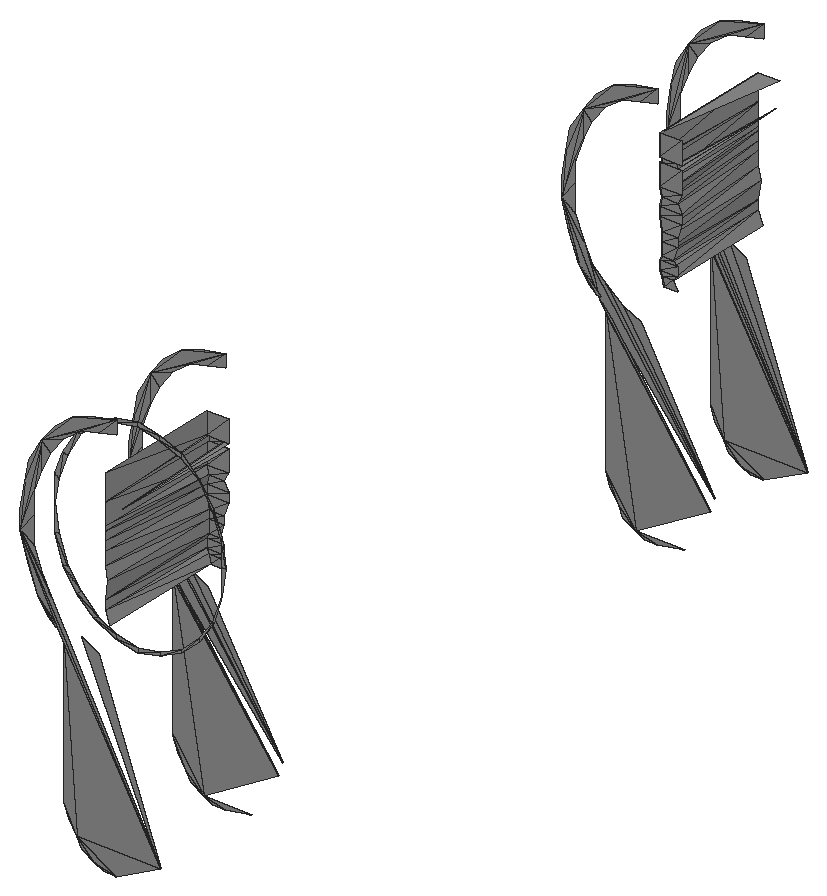
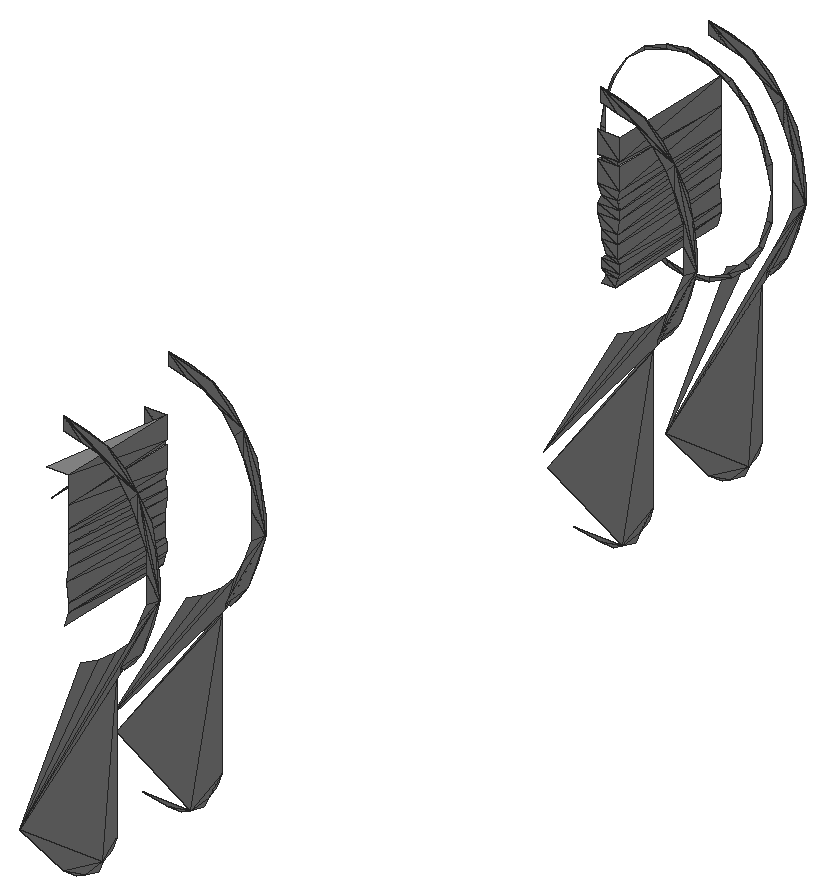
# SketchUp Ruby script. Lengths in inches.
U = 1.inch
M = Sketchup.active_model
def pt(a) = Geom::Point3d.new(a.map { |v| v * U })
def face(e, loops, mat)
  f = e.add_face(loops[0].map { |a| pt(a) })
  loops[1..].each { |l| e.add_face(l.map { |a| pt(a) }).erase! }
  f.material = f.back_material = mat if mat
  f
end
# faces: each face lists its corners as indices into pts; further lists are holes
def faces(e, pts, list, mat = nil) = list.each { |f| face(e, (f[0].is_a?(Array) ? f : [f]).map { |l| l.map { |i| pts[i] } }, mat) }
# xy, xz, yz: faces in a plane at the given z, y or x. An outline is a flat list of corners, or four numbers for a rectangle; further outlines are holes
def ring(l) = l.size == 4 ? [[l[0], l[1]], [l[2], l[1]], [l[2], l[3]], [l[0], l[3]]] : l.each_slice(2).to_a
def flat(e, list, mat, &to3) = list.each { |f| face(e, (f[0].is_a?(Array) ? f : [f]).map { |l| ring(l).map { |u, v| to3.(u, v) } }, mat) }
def xy(e, z, list, mat = nil) = flat(e, list, mat) { |x, y| [x, y, z] }
def xz(e, y, list, mat = nil) = flat(e, list, mat) { |x, z| [x, y, z] }
def yz(e, x, list, mat = nil) = flat(e, list, mat) { |y, z| [x, y, z] }
def lines(e, pts, list) = list.each { |a, b| e.add_line(pt(pts[a]), pt(pts[b])) }
# prism: a flat outline (further loops are holes) pulled along v
def prism(e, loops, v, mat = nil)
  f = face(e, loops, mat); d = Geom::Vector3d.new(v.map { |x| x * U })
  f.pushpull(f.normal.samedirection?(d) ? d.length : -d.length)
end
def box(e, o, s, mat = nil) = prism(e, [[o, [o[0] + s[0], o[1], o[2]], [o[0] + s[0], o[1] + s[1], o[2]], [o[0], o[1] + s[1], o[2]]]], [0, 0, s[2]], mat)
def at(x, y, z, deg = 0) = Geom::Transformation.translation(pt([x, y, z])) * Geom::Transformation.rotation(ORIGIN, Z_AXIS, deg.degrees)
def axes(o, x, y, z) = Geom::Transformation.new([*x, 0, *y, 0, *z, 0, *pt(o).to_a, 1])
def part(name) = M.definitions.add(name)
# library, detail: a bought-in or finely detailed component or shape, given as its bounding box
def library(name, o, s) = part(name).tap { |d| box(d.entities, o, s) }
def detail(e, o, s) = box(e.add_group.entities, o, s)
def put(e, d, t, mat = nil) = e.add_instance(d, t).tap { |i| i.material = mat if mat }
def group(e, t, mat = nil) = e.add_group.tap { |g| g.transformation = t; g.material = mat if mat }.entities
root = M.entities
M.materials.add("Material \#1").color = [140, 140, 140]
xy(root,50.231,[[101.369,117.386,101.417,117.671,101.369,117.671]],"Material \#1")
xz(root,115.821,[[101.393,49.407,101.295,49.462,101.49,49.462],[101.393,49.407,101.338,49.421,101.295,49.462],[101.393,49.407,101.364,49.41,101.338,49.421],[101.338,49.421,101.315,49.439,101.295,49.462],[101.49,49.462,101.172,50.042,101.239,49.931],
  [101.49,49.462,101.263,49.858,101.172,50.042],[101.295,49.462,101.268,49.835,101.268,49.841],[101.295,49.462,101.268,49.841,101.49,49.462],[101.295,49.462,101.271,49.52,101.268,49.835],[101.295,49.462,101.281,49.489,101.271,49.52],
  [101.49,49.462,101.306,49.868,101.348,49.85],[101.271,49.52,101.268,49.554,101.268,49.835],[101.263,49.858,101.26,49.863,101.172,50.042],[101.26,49.863,101.257,49.867,101.172,50.042],[101.257,49.867,101.214,49.919,101.172,50.042],
  [101.257,49.867,101.253,49.872,101.214,49.919],[101.253,49.872,101.232,49.894,101.214,49.919],[101.214,49.919,101.186,49.976,101.172,50.042],[101.214,49.919,101.199,49.947,101.186,49.976],[101.239,49.931,101.172,50.042,101.216,49.974],
  [101.216,49.974,101.172,50.042,101.201,50.023],[101.186,49.976,101.177,50.008,101.172,50.042],[101.201,50.023,101.172,50.042,101.196,50.076],[101.172,50.042,101.17,50.076,101.176,50.137],[101.172,50.042,101.176,50.137,101.219,50.241],
  [101.172,50.042,101.201,50.13,101.196,50.076],[101.172,50.042,101.219,50.241,101.201,50.13],[101.201,50.13,101.219,50.241,101.216,50.179],[101.176,50.137,101.192,50.192,101.219,50.241],[101.216,50.179,101.219,50.241,101.239,50.222],
  [101.239,50.222,101.219,50.241,101.27,50.258],[101.219,50.241,101.253,50.282,101.295,50.313],[101.219,50.241,101.295,50.313,101.393,50.34],[101.219,50.241,101.306,50.285,101.27,50.258],[101.219,50.241,101.393,50.34,101.306,50.285],
  [101.306,50.285,101.393,50.34,101.348,50.303],[101.348,50.303,101.393,50.34,101.393,50.309],[101.295,50.313,101.342,50.333,101.393,50.34]],"Material \#1")
xz(root,115.882,[[101.393,49.844,101.342,49.852,101.393,49.852],[101.393,49.844,101.393,49.852,101.442,49.86],[101.393,49.844,101.442,49.86,101.444,49.852],[101.342,49.852,101.294,49.875,101.344,49.86],[101.342,49.852,101.344,49.86,101.393,49.852],
  [101.444,49.852,101.442,49.86,101.488,49.882],[101.444,49.852,101.488,49.882,101.491,49.875],[101.344,49.86,101.294,49.875,101.298,49.882],[101.294,49.875,101.254,49.912,101.298,49.882],[101.491,49.875,101.488,49.882,101.527,49.918],
  [101.491,49.875,101.527,49.918,101.532,49.912],[101.298,49.882,101.254,49.912,101.258,49.918],[101.254,49.912,101.222,49.96,101.258,49.918],[101.532,49.912,101.527,49.918,101.558,49.964],[101.532,49.912,101.558,49.964,101.563,49.96],
  [101.258,49.918,101.222,49.96,101.228,49.964],[101.222,49.96,101.203,50.016,101.228,49.964],[101.563,49.96,101.558,49.964,101.577,50.018],[101.563,49.96,101.577,50.018,101.583,50.016],[101.228,49.964,101.203,50.016,101.209,50.018],
  [101.203,50.016,101.196,50.076,101.209,50.018],[101.583,50.016,101.577,50.018,101.583,50.076],[101.583,50.016,101.583,50.076,101.59,50.076],[101.209,50.018,101.196,50.076,101.203,50.076],[101.196,50.076,101.203,50.137,101.203,50.076],
  [101.203,50.076,101.203,50.137,101.209,50.135],[101.583,50.076,101.577,50.135,101.59,50.076],[101.59,50.076,101.577,50.135,101.583,50.137],[101.209,50.135,101.203,50.137,101.222,50.193],[101.209,50.135,101.222,50.193,101.228,50.189],
  [101.577,50.135,101.558,50.189,101.583,50.137],[101.583,50.137,101.558,50.189,101.563,50.193],[101.228,50.189,101.222,50.193,101.254,50.241],[101.228,50.189,101.254,50.241,101.258,50.235],[101.558,50.189,101.527,50.235,101.563,50.193],
  [101.563,50.193,101.527,50.235,101.532,50.241],[101.258,50.235,101.254,50.241,101.294,50.278],[101.258,50.235,101.294,50.278,101.298,50.271],[101.527,50.235,101.488,50.271,101.532,50.241],[101.532,50.241,101.488,50.271,101.491,50.278],
  [101.298,50.271,101.294,50.278,101.342,50.301],[101.298,50.271,101.342,50.301,101.344,50.293],[101.488,50.271,101.442,50.293,101.491,50.278],[101.491,50.278,101.442,50.293,101.444,50.301],[101.344,50.293,101.342,50.301,101.393,50.309],
  [101.344,50.293,101.393,50.309,101.393,50.301],[101.442,50.293,101.393,50.301,101.444,50.301],[101.393,50.301,101.393,50.309,101.444,50.301]],"Material \#1")
xz(root,116.097,[[101.384,49.922,101.374,49.945,101.403,49.945],[101.384,49.922,101.403,49.945,101.412,49.922],[101.374,49.945,101.369,49.953,101.408,49.953],[101.374,49.945,101.408,49.953,101.403,49.945],[101.369,49.953,101.369,49.97,101.408,49.97],
  [101.369,49.953,101.408,49.97,101.408,49.953],[101.369,49.97,101.374,49.978,101.403,49.978],[101.369,49.97,101.403,49.978,101.408,49.97],[101.374,49.978,101.374,50.007,101.412,50.007],[101.374,49.978,101.412,50.007,101.403,49.978],
  [101.374,50.007,101.374,50.034,101.412,50.034],[101.374,50.007,101.412,50.034,101.412,50.007],[101.374,50.034,101.367,50.056,101.419,50.056],[101.374,50.034,101.419,50.056,101.412,50.034],[101.367,50.056,101.367,50.078,101.419,50.078],
  [101.367,50.056,101.419,50.078,101.419,50.056],[101.367,50.078,101.374,50.1,101.412,50.1],[101.367,50.078,101.412,50.1,101.419,50.078],[101.374,50.1,101.369,50.115,101.417,50.115],[101.374,50.1,101.417,50.115,101.412,50.1],
  [101.369,50.115,101.369,50.166,101.417,50.166],[101.369,50.115,101.417,50.166,101.417,50.115],[101.369,50.166,101.375,50.169,101.411,50.169],[101.369,50.166,101.411,50.169,101.417,50.166],[101.375,50.169,101.375,50.177,101.411,50.177],
  [101.375,50.169,101.411,50.177,101.411,50.169],[101.375,50.177,101.369,50.181,101.417,50.181],[101.375,50.177,101.417,50.181,101.411,50.177],[101.369,50.181,101.369,50.231,101.417,50.231],[101.369,50.181,101.417,50.231,101.417,50.181]],"Material \#1")
xz(root,116.128,[[101.393,49.407,101.338,49.421,101.364,49.41],[101.393,49.407,101.448,49.421,101.338,49.421],[101.338,49.421,101.268,49.835,101.271,49.52],[101.338,49.421,101.514,49.52,101.268,49.835],[101.338,49.421,101.271,49.52,101.295,49.462],
  [101.338,49.421,101.295,49.462,101.315,49.439],[101.295,49.462,101.271,49.52,101.281,49.489],[101.514,49.52,101.263,49.858,101.265,49.852],[101.514,49.52,101.265,49.852,101.267,49.847],[101.514,49.52,101.267,49.847,101.268,49.841],
  [101.271,49.52,101.268,49.835,101.268,49.554],[101.514,49.52,101.268,49.841,101.268,49.835],[101.517,49.554,101.239,49.931,101.263,49.858],[101.517,49.554,101.27,49.895,101.239,49.931],[101.517,49.554,101.306,49.868,101.27,49.895],
  [101.517,49.554,101.348,49.85,101.306,49.868],[101.263,49.858,101.172,50.042,101.26,49.863],[101.263,49.858,101.216,49.974,101.172,50.042],[101.263,49.858,101.239,49.931,101.216,49.974],[101.26,49.863,101.172,50.042,101.257,49.867],
  [101.257,49.867,101.172,50.042,101.214,49.919],[101.257,49.867,101.214,49.919,101.253,49.872],[101.253,49.872,101.214,49.919,101.232,49.894],[101.214,49.919,101.172,50.042,101.186,49.976],[101.214,49.919,101.186,49.976,101.199,49.947],
  [101.216,49.974,101.201,50.023,101.172,50.042],[101.186,49.976,101.172,50.042,101.177,50.008],[101.201,50.023,101.196,50.076,101.172,50.042],[101.172,50.042,101.176,50.137,101.17,50.076],[101.172,50.042,101.196,50.076,101.201,50.13],
  [101.172,50.042,101.201,50.13,101.216,50.179],[101.172,50.042,101.216,50.179,101.219,50.241],[101.172,50.042,101.219,50.241,101.176,50.137],[101.176,50.137,101.219,50.241,101.192,50.192],[101.216,50.179,101.239,50.222,101.219,50.241],
  [101.239,50.222,101.27,50.258,101.219,50.241],[101.219,50.241,101.27,50.258,101.306,50.285],[101.219,50.241,101.295,50.313,101.253,50.282],[101.219,50.241,101.306,50.285,101.393,50.34],[101.219,50.241,101.393,50.34,101.295,50.313],
  [101.306,50.285,101.348,50.303,101.393,50.34],[101.348,50.303,101.393,50.309,101.393,50.34],[101.295,50.313,101.393,50.34,101.342,50.333]],"Material \#1")
xz(root,117.355,[[101.393,49.407,101.338,49.421,101.448,49.421],[101.393,49.407,101.364,49.41,101.338,49.421],[101.338,49.421,101.268,49.835,101.514,49.52],[101.338,49.421,101.271,49.52,101.268,49.835],[101.338,49.421,101.295,49.462,101.271,49.52],
  [101.338,49.421,101.315,49.439,101.295,49.462],[101.295,49.462,101.281,49.489,101.271,49.52],[101.514,49.52,101.265,49.852,101.263,49.858],[101.514,49.52,101.267,49.847,101.265,49.852],[101.514,49.52,101.268,49.841,101.267,49.847],
  [101.271,49.52,101.268,49.554,101.268,49.835],[101.514,49.52,101.268,49.835,101.268,49.841],[101.517,49.554,101.239,49.931,101.27,49.895],[101.517,49.554,101.263,49.858,101.239,49.931],[101.517,49.554,101.27,49.895,101.306,49.868],
  [101.517,49.554,101.306,49.868,101.348,49.85],[101.263,49.858,101.172,50.042,101.216,49.974],[101.263,49.858,101.26,49.863,101.172,50.042],[101.263,49.858,101.216,49.974,101.239,49.931],[101.26,49.863,101.257,49.867,101.172,50.042],
  [101.257,49.867,101.214,49.919,101.172,50.042],[101.257,49.867,101.253,49.872,101.214,49.919],[101.253,49.872,101.232,49.894,101.214,49.919],[101.214,49.919,101.186,49.976,101.172,50.042],[101.214,49.919,101.199,49.947,101.186,49.976],
  [101.216,49.974,101.172,50.042,101.201,50.023],[101.186,49.976,101.177,50.008,101.172,50.042],[101.201,50.023,101.172,50.042,101.196,50.076],[101.172,50.042,101.17,50.076,101.176,50.137],[101.172,50.042,101.176,50.137,101.219,50.241],
  [101.172,50.042,101.201,50.13,101.196,50.076],[101.172,50.042,101.216,50.179,101.201,50.13],[101.172,50.042,101.219,50.241,101.216,50.179],[101.176,50.137,101.192,50.192,101.219,50.241],[101.216,50.179,101.219,50.241,101.239,50.222],
  [101.239,50.222,101.219,50.241,101.27,50.258],[101.219,50.241,101.253,50.282,101.295,50.313],[101.219,50.241,101.295,50.313,101.393,50.34],[101.219,50.241,101.306,50.285,101.27,50.258],[101.219,50.241,101.393,50.34,101.306,50.285],
  [101.306,50.285,101.393,50.34,101.348,50.303],[101.348,50.303,101.393,50.34,101.393,50.309],[101.295,50.313,101.342,50.333,101.393,50.34]],"Material \#1")
xz(root,117.386,[[101.384,49.922,101.403,49.945,101.374,49.945],[101.384,49.922,101.412,49.922,101.403,49.945],[101.374,49.945,101.408,49.953,101.369,49.953],[101.374,49.945,101.403,49.945,101.408,49.953],[101.369,49.953,101.408,49.953,101.408,49.97],
  [101.369,49.953,101.408,49.97,101.369,49.97],[101.369,49.97,101.403,49.978,101.374,49.978],[101.369,49.97,101.408,49.97,101.403,49.978],[101.374,49.978,101.403,49.978,101.412,50.007],[101.374,49.978,101.412,50.007,101.374,50.007],
  [101.374,50.007,101.412,50.007,101.412,50.034],[101.374,50.007,101.412,50.034,101.374,50.034],[101.374,50.034,101.419,50.056,101.367,50.056],[101.374,50.034,101.412,50.034,101.419,50.056],[101.367,50.056,101.419,50.056,101.419,50.078],
  [101.367,50.056,101.419,50.078,101.367,50.078],[101.367,50.078,101.412,50.1,101.374,50.1],[101.367,50.078,101.419,50.078,101.412,50.1],[101.374,50.1,101.417,50.115,101.369,50.115],[101.374,50.1,101.412,50.1,101.417,50.115],
  [101.369,50.115,101.417,50.115,101.417,50.166],[101.369,50.115,101.417,50.166,101.369,50.166],[101.369,50.166,101.411,50.169,101.375,50.169],[101.369,50.166,101.417,50.166,101.411,50.169],[101.375,50.169,101.411,50.169,101.411,50.177],
  [101.375,50.169,101.411,50.177,101.375,50.177],[101.375,50.177,101.417,50.181,101.369,50.181],[101.375,50.177,101.411,50.177,101.417,50.181],[101.369,50.181,101.417,50.181,101.417,50.231],[101.369,50.181,101.417,50.231,101.369,50.231]],"Material \#1")
xz(root,117.662,[[101.393,49.407,101.295,49.462,101.338,49.421],[101.393,49.407,101.49,49.462,101.295,49.462],[101.393,49.407,101.338,49.421,101.364,49.41],[101.338,49.421,101.295,49.462,101.315,49.439],[101.49,49.462,101.172,50.042,101.263,49.858],
  [101.49,49.462,101.239,49.931,101.172,50.042],[101.49,49.462,101.27,49.895,101.239,49.931],[101.49,49.462,101.263,49.858,101.265,49.852],[101.49,49.462,101.265,49.852,101.267,49.847],[101.49,49.462,101.267,49.847,101.268,49.841],
  [101.295,49.462,101.268,49.835,101.271,49.52],[101.295,49.462,101.268,49.841,101.268,49.835],[101.295,49.462,101.49,49.462,101.268,49.841],[101.49,49.462,101.306,49.868,101.27,49.895],[101.295,49.462,101.271,49.52,101.281,49.489],
  [101.49,49.462,101.348,49.85,101.306,49.868],[101.271,49.52,101.268,49.835,101.268,49.554],[101.263,49.858,101.172,50.042,101.26,49.863],[101.26,49.863,101.172,50.042,101.257,49.867],[101.257,49.867,101.172,50.042,101.214,49.919],
  [101.257,49.867,101.214,49.919,101.253,49.872],[101.253,49.872,101.214,49.919,101.232,49.894],[101.214,49.919,101.172,50.042,101.186,49.976],[101.214,49.919,101.186,49.976,101.199,49.947],[101.239,49.931,101.216,49.974,101.172,50.042],
  [101.216,49.974,101.201,50.023,101.172,50.042],[101.186,49.976,101.172,50.042,101.177,50.008],[101.201,50.023,101.196,50.076,101.172,50.042],[101.172,50.042,101.176,50.137,101.17,50.076],[101.172,50.042,101.196,50.076,101.201,50.13],
  [101.172,50.042,101.201,50.13,101.219,50.241],[101.172,50.042,101.219,50.241,101.176,50.137],[101.201,50.13,101.216,50.179,101.219,50.241],[101.176,50.137,101.219,50.241,101.192,50.192],[101.216,50.179,101.239,50.222,101.219,50.241],
  [101.239,50.222,101.27,50.258,101.219,50.241],[101.219,50.241,101.27,50.258,101.306,50.285],[101.219,50.241,101.295,50.313,101.253,50.282],[101.219,50.241,101.306,50.285,101.393,50.34],[101.219,50.241,101.393,50.34,101.295,50.313],
  [101.306,50.285,101.348,50.303,101.393,50.34],[101.348,50.303,101.393,50.309,101.393,50.34],[101.295,50.313,101.393,50.34,101.342,50.333]],"Material \#1")
yz(root,101.369,[[116.097,50.181,115.812,50.231,116.097,50.231],[117.386,50.181,117.386,50.231,117.671,50.231]],"Material \#1")
yz(root,101.374,[[116.097,49.978,115.812,50.007,116.097,50.007],[117.386,49.978,117.386,50.007,117.671,50.007]],"Material \#1")
p = [[101.369,116.097,49.953],[101.372,115.812,49.949],[101.372,115.812,49.974],[101.372,115.812,49.949],[101.369,116.097,49.953],[101.374,116.097,49.945],
  [101.372,115.812,49.949],[101.374,116.097,49.945],[101.384,116.097,49.922],[101.384,115.812,49.922],[101.372,115.812,49.949],[101.372,117.671,49.974],
  [101.372,117.671,49.949],[101.369,117.386,49.953],[101.372,117.671,49.949],[101.374,117.386,49.945],[101.369,117.386,49.953],[101.372,117.671,49.949],
  [101.384,117.671,49.922],[101.384,117.386,49.922],[101.374,117.386,49.945],[101.372,117.671,49.949],[101.367,115.812,50.067],[101.367,116.097,50.056],
  [101.374,116.097,50.034],[101.369,116.097,49.97],[101.374,116.097,50.034],[101.37,115.812,50.045],[101.367,115.812,50.067],[101.372,115.812,49.974],
  [101.374,116.097,49.978],[101.369,116.097,49.97],[101.37,115.812,50.045],[101.374,116.097,50.034],[101.374,116.097,50.007],[101.374,116.097,50.007],
  [101.374,115.812,50.007],[101.37,115.812,50.045],[101.374,116.097,49.978],[101.372,115.812,49.974],[101.374,115.812,50.007],[101.374,117.386,50.034],
  [101.367,117.386,50.056],[101.367,117.671,50.067],[101.369,117.386,49.97],[101.367,117.671,50.067],[101.37,117.671,50.045],[101.374,117.386,50.034],
  [101.372,117.671,49.974],[101.369,117.386,49.97],[101.374,117.386,49.978],[101.37,117.671,50.045],[101.374,117.671,50.007],[101.374,117.386,50.007],
  [101.374,117.386,50.007],[101.374,117.386,50.034],[101.37,117.671,50.045],[101.374,117.671,50.007],[101.372,117.671,49.974],[101.374,117.386,49.978],
  [101.37,115.812,50.089],[101.367,116.097,50.078],[101.367,116.097,50.056],[101.367,116.097,50.056],[101.367,115.812,50.067],[101.37,115.812,50.089],
  [101.367,116.097,50.078],[101.37,115.812,50.089],[101.372,115.812,50.107],[101.371,115.812,50.17],[101.369,116.097,50.166],[101.369,116.097,50.115],
  [101.369,116.097,50.115],[101.369,115.812,50.119],[101.371,115.812,50.17],[101.372,115.812,50.107],[101.374,116.097,50.1],[101.367,116.097,50.078],
  [101.369,115.812,50.119],[101.369,116.097,50.115],[101.374,116.097,50.1],[101.374,116.097,50.1],[101.372,115.812,50.107],[101.369,115.812,50.119],
  [101.367,117.386,50.056],[101.367,117.386,50.078],[101.37,117.671,50.089],[101.37,117.671,50.089],[101.367,117.671,50.067],[101.367,117.386,50.056],
  [101.372,117.671,50.107],[101.37,117.671,50.089],[101.367,117.386,50.078],[101.369,117.386,50.115],[101.369,117.386,50.166],[101.371,117.671,50.17],
  [101.371,117.671,50.17],[101.369,117.671,50.119],[101.369,117.386,50.115],[101.367,117.386,50.078],[101.374,117.386,50.1],[101.372,117.671,50.107],
  [101.374,117.386,50.1],[101.369,117.386,50.115],[101.369,117.671,50.119],[101.369,117.671,50.119],[101.372,117.671,50.107],[101.374,117.386,50.1],
  [101.369,116.097,50.181],[101.371,115.812,50.17],[101.369,115.812,50.231],[101.414,115.812,50.175],[101.417,116.097,50.166],[101.411,116.097,50.169],
  [101.371,115.812,50.17],[101.375,116.097,50.177],[101.375,116.097,50.169],[101.371,115.812,50.17],[101.369,116.097,50.181],[101.371,115.812,50.17],
  [101.369,116.097,50.166],[101.414,115.812,50.175],[101.411,116.097,50.177],[101.417,116.097,50.181],[101.414,115.812,50.175],[101.369,117.671,50.231],
  [101.371,117.671,50.17],[101.369,117.386,50.181],[101.414,117.671,50.175],[101.411,117.386,50.169],[101.417,117.386,50.166],[101.371,117.671,50.17],
  [101.375,117.386,50.169],[101.375,117.386,50.177],[101.371,117.671,50.17],[101.369,117.386,50.181],[101.371,117.671,50.17],[101.369,117.386,50.166],
  [101.414,117.671,50.175],[101.417,117.386,50.181],[101.411,117.386,50.177],[101.414,117.671,50.175]]
faces(root,p,[[0,1,2],[3,4,5],[6,7,8],[8,9,10],[11,12,13],[14,15,16],[17,18,19],[19,20,21],
  [22,23,24],[2,25,0],[26,27,28],[29,30,31],[32,33,34],[35,36,37],[38,39,40],[41,42,43],
  [13,44,11],[45,46,47],[48,49,50],[51,52,53],[54,55,56],[57,58,59],[60,61,62],[63,64,65],
  [66,67,68],[69,70,71],[72,73,74],[75,76,77],[78,79,80],[81,82,83],[84,85,86],[87,88,89],
  [90,91,92],[93,94,95],[96,97,98],[99,100,101],[102,103,104],[105,106,107],[108,109,110],[111,112,113],
  [114,115,116],[117,118,115],[119,116,120],[121,122,123],[124,113,122],[125,126,127],[128,129,130],[131,132,133],
  [134,133,135],[136,137,132],[138,139,140],[141,140,129]],"Material \#1")
